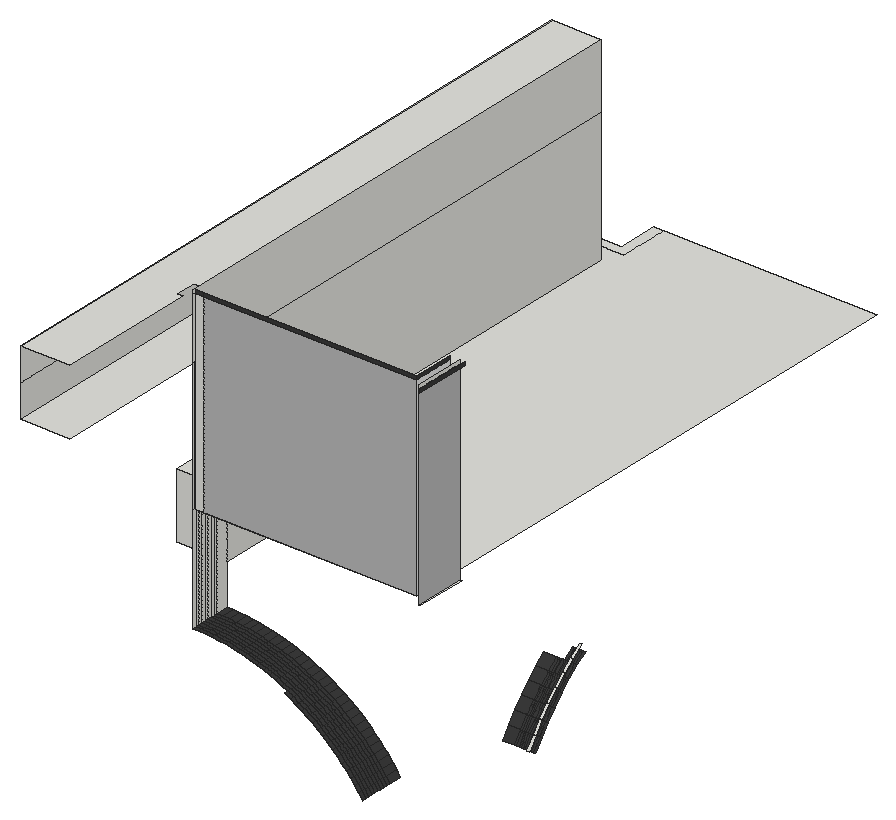
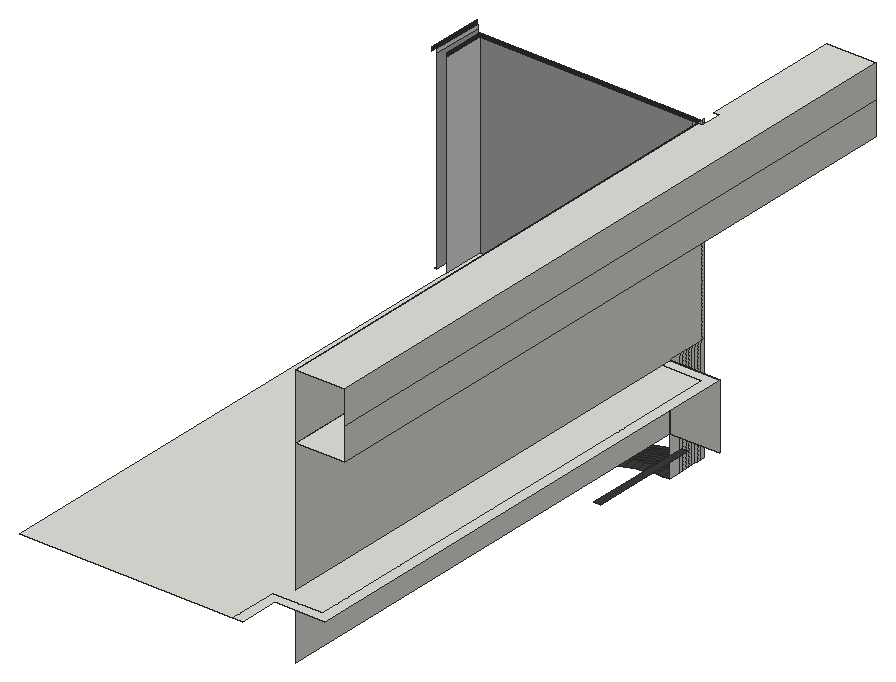
# SketchUp Ruby script. Lengths in inches.
U = 1.inch
M = Sketchup.active_model
def pt(a) = Geom::Point3d.new(a.map { |v| v * U })
def face(e, loops, mat)
  f = e.add_face(loops[0].map { |a| pt(a) })
  loops[1..].each { |l| e.add_face(l.map { |a| pt(a) }).erase! }
  f.material = f.back_material = mat if mat
  f
end
# faces: each face lists its corners as indices into pts; further lists are holes
def faces(e, pts, list, mat = nil) = list.each { |f| face(e, (f[0].is_a?(Array) ? f : [f]).map { |l| l.map { |i| pts[i] } }, mat) }
# xy, xz, yz: faces in a plane at the given z, y or x. An outline is a flat list of corners, or four numbers for a rectangle; further outlines are holes
def ring(l) = l.size == 4 ? [[l[0], l[1]], [l[2], l[1]], [l[2], l[3]], [l[0], l[3]]] : l.each_slice(2).to_a
def flat(e, list, mat, &to3) = list.each { |f| face(e, (f[0].is_a?(Array) ? f : [f]).map { |l| ring(l).map { |u, v| to3.(u, v) } }, mat) }
def xy(e, z, list, mat = nil) = flat(e, list, mat) { |x, y| [x, y, z] }
def xz(e, y, list, mat = nil) = flat(e, list, mat) { |x, z| [x, y, z] }
def yz(e, x, list, mat = nil) = flat(e, list, mat) { |y, z| [x, y, z] }
def lines(e, pts, list) = list.each { |a, b| e.add_line(pt(pts[a]), pt(pts[b])) }
# prism: a flat outline (further loops are holes) pulled along v
def prism(e, loops, v, mat = nil)
  f = face(e, loops, mat); d = Geom::Vector3d.new(v.map { |x| x * U })
  f.pushpull(f.normal.samedirection?(d) ? d.length : -d.length)
end
def box(e, o, s, mat = nil) = prism(e, [[o, [o[0] + s[0], o[1], o[2]], [o[0] + s[0], o[1] + s[1], o[2]], [o[0], o[1] + s[1], o[2]]]], [0, 0, s[2]], mat)
def at(x, y, z, deg = 0) = Geom::Transformation.translation(pt([x, y, z])) * Geom::Transformation.rotation(ORIGIN, Z_AXIS, deg.degrees)
def axes(o, x, y, z) = Geom::Transformation.new([*x, 0, *y, 0, *z, 0, *pt(o).to_a, 1])
def part(name) = M.definitions.add(name)
# library, detail: a bought-in or finely detailed component or shape, given as its bounding box
def library(name, o, s) = part(name).tap { |d| box(d.entities, o, s) }
def detail(e, o, s) = box(e.add_group.entities, o, s)
def put(e, d, t, mat = nil) = e.add_instance(d, t).tap { |i| i.material = mat if mat }
def group(e, t, mat = nil) = e.add_group.tap { |g| g.transformation = t; g.material = mat if mat }.entities
root = M.entities
M.materials.add("[Color M07]").color = [58, 58, 58]
M.materials.add("[Mirror 01]").color = [185, 185, 185]
M.materials.add("[Mirror 02]").color = [229, 229, 229]
xy(root,336.73,[[150.22,125.93,151.47,146.03]],"[Color M07]")
xy(root,349.6875,[[196.96,115.71,197.34,124.96],[154.46,117.49,156.24,117.49,156.24,126.74,147.05,126.74,147.05,213.44,156.24,213.44,156.24,222.44,154.46,222.44,154.46,215.22,145.27,215.22,145.27,124.96,154.46,124.96],[156.24,117.49,195.18,117.49,195.18,222.44,156.24,222.44,156.24,213.44,147.05,213.44,147.05,126.74,156.24,126.74]])
xy(root,373.6875,[[145.46,88.96,154.46,210.47]])
xy(root,385.6875,[[145.46,88.96,154.46,88.96,154.46,114.76,153.51,114.76,153.51,118.4375,154.46,118.4375,154.46,210.47,145.46,210.47]])
xz(root,117.49,[[154.46,349.6875,156.24,385.0625]])
xz(root,117.49,[[154.46,385.0625,156.24,385.6875],[156.24,385.0625,195.18,385.6875]],"[Color M07]")
xz(root,117.49,[[156.24,349.6875,195.18,385.0625]],"[Mirror 01]")
xz(root,124.96,[[145.27,337.6875,154.46,349.6875]])
yz(root,145.46,[[88.96,373.6875,210.47,379.6875],[88.96,379.6875,210.47,385.6875]])
yz(root,154.46,[[117.08,330.25,117.77,349.6875],[117.77,330.25,118.46,349.6875],[118.46,330.25,119.14,349.6875],[119.14,330.25,119.83,349.6875],[119.83,330.25,120.52,349.6875],
  [120.52,330.25,121.21,349.6875],[121.21,330.25,121.89,349.6875],[121.89,330.25,122.58,349.6875],[122.58,330.25,124.96,349.6875],[124.96,337.6875,210.47,337.6875,210.47,373.6875,117.49,373.6875,117.49,349.6875,124.96,349.6875],
  [117.08,349.6875,117.49,373.6875],[117.08,373.6875,117.49,385.0625],[117.49,373.6875,210.47,385.6875],[117.08,385.0625,117.49,385.6875]])
yz(root,195.18,[[117.49,385.0625,124.96,385.6875]],"[Color M07]")
yz(root,195.18,[[117.49,349.6875,124.96,385.0625]],"[Mirror 02]")
yz(root,196.96,[[115.71,385.0625,124.96,385.6875]])
yz(root,196.96,[[115.71,349.6875,124.96,385.0625]],"[Mirror 01]")
yz(root,197.91,[[114.76,385.0625,124.96,385.6875]],"[Color M07]")
p = [[185.43,116.39,314.47],[185.43,117.08,314.47],[186.12,117.08,313.49],[186.12,116.39,313.49],[185.43,117.77,314.47],[186.12,117.77,313.49],
  [185.43,118.46,314.47],[186.12,118.46,313.49],[185.43,119.14,314.47],[186.12,119.14,313.49],[185.43,119.83,314.47],[186.12,119.83,313.49],
  [185.43,120.52,314.47],[186.12,120.52,313.49],[185.43,121.21,314.47],[186.12,121.21,313.49],[185.43,121.89,314.47],[186.12,121.89,313.49],
  [185.43,122.58,314.47],[186.12,122.58,313.49],[186.12,124.96,313.49],[185.43,124.96,314.47],[190.96,143.68,315.55],[193.21,143.68,315.55],
  [193.21,142.38,313.61],[190.96,142.38,313.61],[193.59,142.38,313.61],[193.59,143.68,315.55],[193.96,142.38,313.61],[193.96,143.68,315.55],
  [194.34,142.38,313.61],[194.34,143.68,315.55],[194.71,142.38,313.61],[194.71,143.68,315.55],[195.09,142.38,313.61],[195.09,143.68,315.55],
  [195.46,142.38,313.61],[195.46,143.68,315.55],[195.84,142.38,313.61],[195.84,143.68,315.55],[196.21,142.38,313.61],[196.21,143.68,315.55],
  [196.59,142.38,313.61],[196.59,143.68,315.55],[196.96,142.38,313.61],[196.96,143.68,315.55],[184.71,116.39,315.43],[184.71,117.08,315.43],
  [184.71,117.77,315.43],[184.71,118.46,315.43],[184.71,119.14,315.43],[184.71,119.83,315.43],[184.71,120.52,315.43],[184.71,121.21,315.43],
  [184.71,121.89,315.43],[184.71,122.58,315.43],[184.71,124.96,315.43],[196.96,140.44,314.82],[196.96,141.83,316.88],[197.34,141.83,316.88],
  [197.34,140.44,314.82],[183.96,116.39,316.37],[183.96,117.08,316.37],[183.96,117.77,316.37],[183.96,118.46,316.37],[183.96,119.14,316.37],
  [183.96,119.83,316.37],[183.96,120.52,316.37],[183.96,121.21,316.37],[183.96,121.89,316.37],[183.96,122.58,316.37],[183.96,124.96,316.37],
  [190.96,145.1,317.42],[193.21,145.1,317.42],[193.59,145.1,317.42],[193.96,145.1,317.42],[194.34,145.1,317.42],[194.71,145.1,317.42],
  [195.09,145.1,317.42],[195.46,145.1,317.42],[195.84,145.1,317.42],[196.21,145.1,317.42],[196.59,145.1,317.42],[196.96,145.1,317.42],
  [183.18,116.39,317.28],[183.18,117.08,317.28],[183.18,117.77,317.28],[183.18,118.46,317.28],[183.18,119.14,317.28],[183.18,119.83,317.28],
  [183.18,120.52,317.28],[183.18,121.21,317.28],[183.18,121.89,317.28],[183.18,122.58,317.28],[183.18,124.96,317.28],[196.96,143.33,318.85],
  [197.34,143.33,318.85],[182.37,116.39,318.17],[182.37,117.08,318.17],[182.37,117.77,318.17],[182.37,118.46,318.17],[182.37,119.14,318.17],
  [182.37,119.83,318.17],[182.37,120.52,318.17],[182.37,121.21,318.17],[182.37,121.89,318.17],[182.37,122.58,318.17],[182.37,124.96,318.17],
  [190.96,146.63,319.19],[193.21,146.63,319.19],[193.59,146.63,319.19],[193.96,146.63,319.19],[194.34,146.63,319.19],[194.71,146.63,319.19],
  [195.09,146.63,319.19],[195.46,146.63,319.19],[195.84,146.63,319.19],[196.21,146.63,319.19],[196.59,146.63,319.19],[196.96,146.63,319.19],
  [181.53,116.39,319.04],[181.53,117.08,319.04],[181.53,117.77,319.04],[181.53,118.46,319.04],[181.53,119.14,319.04],[181.53,119.83,319.04],
  [181.53,120.52,319.04],[181.53,121.21,319.04],[181.53,121.89,319.04],[181.53,122.58,319.04],[181.53,124.96,319.04],[196.96,144.94,320.73],
  [197.34,144.94,320.73],[180.67,116.39,319.875],[180.67,117.08,319.875],[180.67,117.77,319.875],[180.67,118.46,319.875],[180.67,119.14,319.875],
  [180.67,119.83,319.875],[180.67,120.52,319.875],[180.67,121.21,319.875],[180.67,121.89,319.875],[180.67,122.58,319.875],[180.67,124.96,319.875],
  [190.96,148.26,320.88],[193.21,148.26,320.88],[193.59,148.26,320.88],[193.96,148.26,320.88],[194.34,148.26,320.88],[194.71,148.26,320.88],
  [195.09,148.26,320.88],[195.46,148.26,320.88],[195.84,148.26,320.88],[196.21,148.26,320.88],[196.59,148.26,320.88],[196.96,148.26,320.88],
  [179.78,116.39,320.68],[179.78,117.08,320.68],[179.78,117.77,320.68],[179.78,118.46,320.68],[179.78,119.14,320.68],[179.78,119.83,320.68],
  [179.78,120.52,320.68],[179.78,121.21,320.68],[179.78,121.89,320.68],[179.78,122.58,320.68],[179.78,124.96,320.68],[178.86,116.39,321.46],
  [178.86,117.08,321.46],[178.86,117.77,321.46],[178.86,118.46,321.46],[178.86,119.14,321.46],[178.86,119.83,321.46],[178.86,120.52,321.46],
  [178.86,121.21,321.46],[178.86,121.89,321.46],[178.86,122.58,321.46],[178.86,124.96,321.46],[196.96,146.67,322.51],[197.34,146.67,322.51],
  [190.96,149.99,322.46],[193.21,149.99,322.46],[193.59,149.99,322.46],[193.96,149.99,322.46],[194.34,149.99,322.46],[194.71,149.99,322.46],
  [195.09,149.99,322.46],[195.46,149.99,322.46],[195.84,149.99,322.46],[196.21,149.99,322.46],[196.59,149.99,322.46],[196.96,149.99,322.46],
  [177.92,116.39,322.22],[177.92,117.08,322.22],[177.92,117.77,322.22],[177.92,118.46,322.22],[177.92,119.14,322.22],[177.92,119.83,322.22],
  [177.92,120.52,322.22],[177.92,121.21,322.22],[177.92,121.89,322.22],[177.92,122.58,322.22],[177.92,124.96,322.22],[176.96,116.39,322.9375],
  [176.96,117.08,322.9375],[176.96,117.77,322.9375],[176.96,118.46,322.9375],[176.96,119.14,322.9375],[176.96,119.83,322.9375],[176.96,120.52,322.9375],
  [176.96,121.21,322.9375],[176.96,121.89,322.9375],[176.96,122.58,322.9375],[176.96,124.96,322.9375],[196.96,148.5,324.1875],[197.34,148.5,324.1875],
  [190.96,151.81,323.9375],[193.21,151.81,323.9375],[193.59,151.81,323.9375],[193.96,151.81,323.9375],[194.34,151.81,323.9375],[194.71,151.81,323.9375],
  [195.09,151.81,323.9375],[195.46,151.81,323.9375],[195.84,151.81,323.9375],[196.21,151.81,323.9375],[196.59,151.81,323.9375],[196.96,151.81,323.9375],
  [175.98,116.39,323.63],[175.98,117.08,323.63],[175.98,117.77,323.63],[175.98,118.46,323.63],[175.98,119.14,323.63],[175.98,119.83,323.63],
  [175.98,120.52,323.63],[175.98,121.21,323.63],[175.98,121.89,323.63],[175.98,122.58,323.63],[175.98,124.96,323.63],[174.97,116.39,324.29],
  [174.97,117.08,324.29],[174.97,117.77,324.29],[174.97,118.46,324.29],[174.97,119.14,324.29],[174.97,119.83,324.29],[174.97,120.52,324.29],
  [174.97,121.21,324.29],[174.97,121.89,324.29],[174.97,122.58,324.29],[174.97,124.96,324.29],[194.71,153.71,325.31],[195.09,153.71,325.31],
  [195.46,153.71,325.31],[195.84,153.71,325.31],[196.21,153.71,325.31],[196.59,153.71,325.31],[196.96,153.71,325.31],[196.96,150.42,325.75],
  [197.34,150.42,325.75],[173.95,116.39,324.92],[173.95,117.08,324.92],[173.95,117.77,324.92],[173.95,118.46,324.92],[173.95,119.14,324.92],
  [173.95,119.83,324.92],[173.95,120.52,324.92],[173.95,121.21,324.92],[173.95,121.89,324.92],[173.95,122.58,324.92],[173.95,124.96,324.92],
  [172.9,116.39,325.51],[172.9,117.08,325.51],[172.9,117.77,325.51],[172.9,118.46,325.51],[172.9,119.14,325.51],[172.9,119.83,325.51],
  [172.9,120.52,325.51],[172.9,121.21,325.51],[172.9,121.89,325.51],[172.9,122.58,325.51],[172.9,124.96,325.51],[171.84,116.39,326.08],
  [171.84,117.08,326.08],[171.84,117.77,326.08],[171.84,118.46,326.08],[171.84,119.14,326.08],[171.84,119.83,326.08],[171.84,120.52,326.08],
  [171.84,121.21,326.08],[171.84,121.89,326.08],[171.84,122.58,326.08],[171.84,124.96,326.08],[196.96,152.43,327.2],[197.34,152.43,327.2],
  [170.76,117.08,326.61],[170.76,117.77,326.61],[170.76,118.46,326.61],[170.76,119.14,326.61],[170.76,119.83,326.61],[170.76,120.52,326.61],
  [170.76,121.21,326.61],[170.76,121.89,326.61],[170.76,122.58,326.61],[170.76,124.96,326.61],[169.66,117.08,327.1],[169.66,117.77,327.1],
  [169.66,118.46,327.1],[169.66,119.14,327.1],[169.66,119.83,327.1],[169.66,120.52,327.1],[169.66,121.21,327.1],[169.66,121.89,327.1],
  [169.66,122.58,327.1],[169.66,124.96,327.1],[168.55,117.08,327.5625],[168.55,117.77,327.5625],[168.55,118.46,327.5625],[168.55,119.14,327.5625],
  [168.55,119.83,327.5625],[168.55,120.52,327.5625],[168.55,121.21,327.5625],[168.55,121.89,327.5625],[168.55,122.58,327.5625],[168.55,124.96,327.5625],
  [167.43,117.08,327.99],[167.43,117.77,327.99],[167.43,118.46,327.99],[167.43,119.14,327.99],[167.43,119.83,327.99],[167.43,120.52,327.99],
  [167.43,121.21,327.99],[167.43,121.89,327.99],[167.43,122.58,327.99],[167.43,124.96,327.99],[166.29,117.08,328.375],[166.29,117.77,328.375],
  [166.29,118.46,328.375],[166.29,119.14,328.375],[166.29,119.83,328.375],[166.29,120.52,328.375],[166.29,121.21,328.375],[166.29,121.89,328.375],
  [166.29,122.58,328.375],[166.29,124.96,328.375],[165.14,117.08,328.73],[165.14,117.77,328.73],[165.14,118.46,328.73],[165.14,119.14,328.73],
  [165.14,119.83,328.73],[165.14,120.52,328.73],[165.14,121.21,328.73],[165.14,121.89,328.73],[165.14,122.58,328.73],[165.14,124.96,328.73],
  [163.98,117.08,329.05],[163.98,117.77,329.05],[163.98,118.46,329.05],[163.98,119.14,329.05],[163.98,119.83,329.05],[163.98,120.52,329.05],
  [163.98,121.21,329.05],[163.98,121.89,329.05],[163.98,122.58,329.05],[163.98,124.96,329.05],[162.8125,117.08,329.33],[162.8125,117.77,329.33],
  [162.8125,118.46,329.33],[162.8125,119.14,329.33],[162.8125,119.83,329.33],[162.8125,120.52,329.33],[162.8125,121.21,329.33],[162.8125,121.89,329.33],
  [162.8125,122.58,329.33],[162.8125,124.96,329.33],[161.63,117.08,329.57],[161.63,117.77,329.57],[161.63,118.46,329.57],[161.63,119.14,329.57],
  [161.63,119.83,329.57],[161.63,120.52,329.57],[161.63,121.21,329.57],[161.63,121.89,329.57],[161.63,122.58,329.57],[161.63,124.96,329.57],
  [160.45,117.08,329.78],[160.45,117.77,329.78],[160.45,118.46,329.78],[160.45,119.14,329.78],[160.45,119.83,329.78],[160.45,120.52,329.78],
  [160.45,121.21,329.78],[160.45,121.89,329.78],[160.45,122.58,329.78],[160.45,124.96,329.78],[159.26,117.08,329.95],[159.26,117.77,329.95],
  [159.26,118.46,329.95],[159.26,119.14,329.95],[159.26,119.83,329.95],[159.26,120.52,329.95],[159.26,121.21,329.95],[159.26,121.89,329.95],
  [159.26,122.58,329.95],[159.26,124.96,329.95],[158.0625,117.08,330.08],[158.0625,117.77,330.08],[158.0625,118.46,330.08],[158.0625,119.14,330.08],
  [158.0625,119.83,330.08],[158.0625,120.52,330.08],[158.0625,121.21,330.08],[158.0625,121.89,330.08],[158.0625,122.58,330.08],[158.0625,124.96,330.08],
  [156.86,117.08,330.17],[156.86,117.77,330.17],[156.86,118.46,330.17],[156.86,119.14,330.17],[156.86,119.83,330.17],[156.86,120.52,330.17],
  [156.86,121.21,330.17],[156.86,121.89,330.17],[156.86,122.58,330.17],[156.86,124.96,330.17],[154.46,117.08,330.25],[154.46,117.77,330.25],
  [155.66,117.77,330.23],[155.66,117.08,330.23],[154.46,118.46,330.25],[155.66,118.46,330.23],[154.46,119.14,330.25],[155.66,119.14,330.23],
  [154.46,119.83,330.25],[155.66,119.83,330.23],[154.46,120.52,330.25],[155.66,120.52,330.23],[154.46,121.21,330.25],[155.66,121.21,330.23],
  [154.46,121.89,330.25],[155.66,121.89,330.23],[154.46,122.58,330.25],[155.66,122.58,330.23],[155.66,124.96,330.23],[154.46,124.96,330.25]]
faces(root,p,[[0,1,2,3],[1,4,5,2],[4,6,7,5],[6,8,9,7],[8,10,11,9],[10,12,13,11],[12,14,15,13],[14,16,17,15],
  [16,18,19,17],[20,19,18,21],[22,23,24,25],[26,24,23,27],[28,26,27,29],[30,28,29,31],[32,30,31,33],[34,32,33,35],
  [36,34,35,37],[38,36,37,39],[40,38,39,41],[42,40,41,43],[44,42,43,45],[46,47,1,0],[47,48,4,1],[48,49,6,4],
  [49,50,8,6],[50,51,10,8],[51,52,12,10],[52,53,14,12],[53,54,16,14],[54,55,18,16],[21,18,55,56],[61,62,47,46],
  [62,63,48,47],[63,64,49,48],[64,65,50,49],[65,66,51,50],[66,67,52,51],[67,68,53,52],[68,69,54,53],[69,70,55,54],
  [56,55,70,71],[72,73,23,22],[27,23,73,74],[29,27,74,75],[31,29,75,76],[33,31,76,77],[35,33,77,78],[37,35,78,79],
  [39,37,79,80],[41,39,80,81],[43,41,81,82],[45,43,82,83],[84,85,62,61],[85,86,63,62],[86,87,64,63],[87,88,65,64],
  [88,89,66,65],[89,90,67,66],[90,91,68,67],[91,92,69,68],[92,93,70,69],[71,70,93,94],[97,98,85,84],[98,99,86,85],
  [99,100,87,86],[100,101,88,87],[101,102,89,88],[102,103,90,89],[103,104,91,90],[104,105,92,91],[105,106,93,92],[94,93,106,107],
  [108,109,73,72],[74,73,109,110],[75,74,110,111],[76,75,111,112],[77,76,112,113],[78,77,113,114],[79,78,114,115],[80,79,115,116],
  [81,80,116,117],[82,81,117,118],[83,82,118,119],[120,121,98,97],[121,122,99,98],[122,123,100,99],[123,124,101,100],[124,125,102,101],
  [125,126,103,102],[126,127,104,103],[127,128,105,104],[128,129,106,105],[107,106,129,130],[133,134,121,120],[134,135,122,121],[135,136,123,122],
  [136,137,124,123],[137,138,125,124],[138,139,126,125],[139,140,127,126],[140,141,128,127],[141,142,129,128],[130,129,142,143],[144,145,109,108],
  [110,109,145,146],[111,110,146,147],[112,111,147,148],[113,112,148,149],[114,113,149,150],[115,114,150,151],[116,115,151,152],[117,116,152,153],
  [118,117,153,154],[119,118,154,155],[156,157,134,133],[157,158,135,134],[158,159,136,135],[159,160,137,136],[160,161,138,137],[161,162,139,138],
  [162,163,140,139],[163,164,141,140],[164,165,142,141],[143,142,165,166],[167,168,157,156],[168,169,158,157],[169,170,159,158],[170,171,160,159],
  [171,172,161,160],[172,173,162,161],[173,174,163,162],[174,175,164,163],[175,176,165,164],[166,165,176,177],[180,181,145,144],[146,145,181,182],
  [147,146,182,183],[148,147,183,184],[149,148,184,185],[150,149,185,186],[151,150,186,187],[152,151,187,188],[153,152,188,189],[154,153,189,190],
  [155,154,190,191],[192,193,168,167],[193,194,169,168],[194,195,170,169],[195,196,171,170],[196,197,172,171],[197,198,173,172],[198,199,174,173],
  [199,200,175,174],[200,201,176,175],[177,176,201,202],[203,204,193,192],[204,205,194,193],[205,206,195,194],[206,207,196,195],[207,208,197,196],
  [208,209,198,197],[209,210,199,198],[210,211,200,199],[211,212,201,200],[202,201,212,213],[216,217,181,180],[182,181,217,218],[183,182,218,219],
  [184,183,219,220],[185,184,220,221],[186,185,221,222],[187,186,222,223],[188,187,223,224],[189,188,224,225],[190,189,225,226],[191,190,226,227],
  [228,229,204,203],[229,230,205,204],[230,231,206,205],[231,232,207,206],[232,233,208,207],[233,234,209,208],[234,235,210,209],[235,236,211,210],
  [236,237,212,211],[213,212,237,238],[239,240,229,228],[240,241,230,229],[241,242,231,230],[242,243,232,231],[243,244,233,232],[244,245,234,233],
  [245,246,235,234],[246,247,236,235],[247,248,237,236],[238,237,248,249],[222,221,250,251],[223,222,251,252],[224,223,252,253],[225,224,253,254],
  [226,225,254,255],[227,226,255,256],[259,260,240,239],[260,261,241,240],[261,262,242,241],[262,263,243,242],[263,264,244,243],[264,265,245,244],
  [265,266,246,245],[266,267,247,246],[267,268,248,247],[249,248,268,269],[270,271,260,259],[271,272,261,260],[272,273,262,261],[273,274,263,262],
  [274,275,264,263],[275,276,265,264],[276,277,266,265],[277,278,267,266],[278,279,268,267],[269,268,279,280],[281,282,271,270],[282,283,272,271],
  [283,284,273,272],[284,285,274,273],[285,286,275,274],[286,287,276,275],[287,288,277,276],[288,289,278,277],[289,290,279,278],[280,279,290,291],
  [294,295,283,282],[295,296,284,283],[296,297,285,284],[297,298,286,285],[298,299,287,286],[299,300,288,287],[300,301,289,288],[301,302,290,289],
  [291,290,302,303],[304,305,295,294],[305,306,296,295],[306,307,297,296],[307,308,298,297],[308,309,299,298],[309,310,300,299],[310,311,301,300],
  [311,312,302,301],[303,302,312,313],[314,315,305,304],[315,316,306,305],[316,317,307,306],[317,318,308,307],[318,319,309,308],[319,320,310,309],
  [320,321,311,310],[321,322,312,311],[313,312,322,323],[324,325,315,314],[325,326,316,315],[326,327,317,316],[327,328,318,317],[328,329,319,318],
  [329,330,320,319],[330,331,321,320],[331,332,322,321],[323,322,332,333],[334,335,325,324],[335,336,326,325],[336,337,327,326],[337,338,328,327],
  [338,339,329,328],[339,340,330,329],[340,341,331,330],[341,342,332,331],[333,332,342,343],[344,345,335,334],[345,346,336,335],[346,347,337,336],
  [347,348,338,337],[348,349,339,338],[349,350,340,339],[350,351,341,340],[351,352,342,341],[343,342,352,353],[354,355,345,344],[355,356,346,345],
  [356,357,347,346],[357,358,348,347],[358,359,349,348],[359,360,350,349],[360,361,351,350],[361,362,352,351],[353,352,362,363],[364,365,355,354],
  [365,366,356,355],[366,367,357,356],[367,368,358,357],[368,369,359,358],[369,370,360,359],[370,371,361,360],[371,372,362,361],[363,362,372,373],
  [374,375,365,364],[375,376,366,365],[376,377,367,366],[377,378,368,367],[378,379,369,368],[379,380,370,369],[380,381,371,370],[381,382,372,371],
  [373,372,382,383],[384,385,375,374],[385,386,376,375],[386,387,377,376],[387,388,378,377],[388,389,379,378],[389,390,380,379],[390,391,381,380],
  [391,392,382,381],[383,382,392,393],[394,395,385,384],[395,396,386,385],[396,397,387,386],[397,398,388,387],[398,399,389,388],[399,400,390,389],
  [400,401,391,390],[401,402,392,391],[393,392,402,403],[404,405,395,394],[405,406,396,395],[406,407,397,396],[407,408,398,397],[408,409,399,398],
  [409,410,400,399],[410,411,401,400],[411,412,402,401],[403,402,412,413],[414,415,405,404],[415,416,406,405],[416,417,407,406],[417,418,408,407],
  [418,419,409,408],[419,420,410,409],[420,421,411,410],[421,422,412,411],[413,412,422,423],[424,425,426,427],[427,426,415,414],[425,428,429,426],
  [426,429,416,415],[428,430,431,429],[429,431,417,416],[430,432,433,431],[431,433,418,417],[432,434,435,433],[433,435,419,418],[434,436,437,435],
  [435,437,420,419],[436,438,439,437],[437,439,421,420],[438,440,441,439],[439,441,422,421],[442,441,440,443],[423,422,441,442]],"[Color M07]")
faces(root,p,[[57,58,59,60],[58,95,96,59],[95,131,132,96],[131,178,179,132],[178,214,215,179],[214,257,258,215],[257,292,293,258]])
